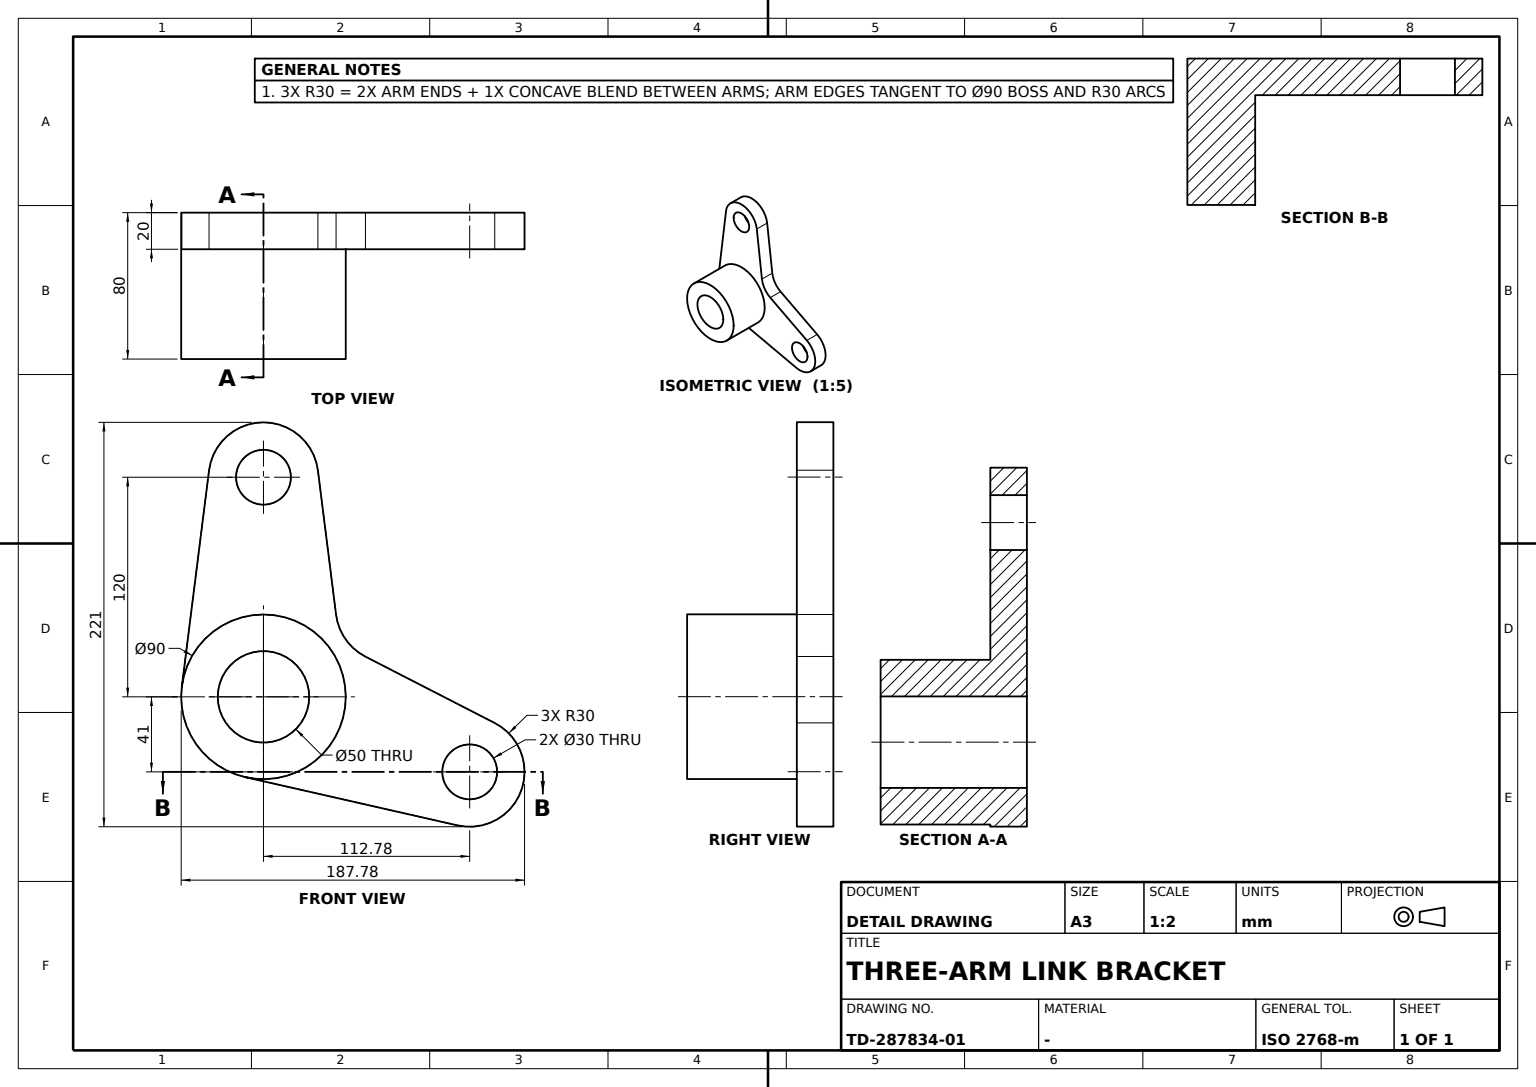
ISO-10303-21;
HEADER;
FILE_DESCRIPTION((''),'2;1');
FILE_NAME('','',(''),(''),'','','');
FILE_SCHEMA(('AUTOMOTIVE_DESIGN'));
ENDSEC;
DATA;
#1=APPLICATION_CONTEXT('');
#2=PRODUCT_CONTEXT('',#1,'mechanical');
#3=PRODUCT('','','',(#2));
#4=PRODUCT_DEFINITION_FORMATION('','',#3);
#5=PRODUCT_DEFINITION_CONTEXT('',#1,'design');
#6=PRODUCT_DEFINITION('','',#4,#5);
#7=PRODUCT_DEFINITION_SHAPE('','',#6);
#8=(LENGTH_UNIT()NAMED_UNIT(*)SI_UNIT(.MILLI.,.METRE.));
#9=(NAMED_UNIT(*)PLANE_ANGLE_UNIT()SI_UNIT($,.RADIAN.));
#10=(NAMED_UNIT(*)SI_UNIT($,.STERADIAN.)SOLID_ANGLE_UNIT());
#11=UNCERTAINTY_MEASURE_WITH_UNIT(LENGTH_MEASURE(1.E-05),#8,'distance_accuracy_value','');
#12=(GEOMETRIC_REPRESENTATION_CONTEXT(3)GLOBAL_UNCERTAINTY_ASSIGNED_CONTEXT((#11))GLOBAL_UNIT_ASSIGNED_CONTEXT((#8,#9,#10))REPRESENTATION_CONTEXT('',''));
#13=CARTESIAN_POINT('',(20.,45.,0.));
#14=VERTEX_POINT('',#13);
#15=CARTESIAN_POINT('',(20.,-44.647053,5.625));
#16=VERTEX_POINT('',#15);
#17=CARTESIAN_POINT('',(20.,0.,0.));
#18=DIRECTION('',(1.,0.,0.));
#19=DIRECTION('',(0.,1.,0.));
#20=AXIS2_PLACEMENT_3D('',#17,#18,#19);
#21=CIRCLE('',#20,45.);
#22=EDGE_CURVE('',#14,#16,#21,.T.);
#23=ORIENTED_EDGE('',*,*,#22,.T.);
#24=CARTESIAN_POINT('',(80.,-44.647053,5.625));
#25=VERTEX_POINT('',#24);
#26=CARTESIAN_POINT('',(40.,-44.647053,5.625));
#27=VECTOR('',#18,1000.);
#28=LINE('',#26,#27);
#29=EDGE_CURVE('',#16,#25,#28,.T.);
#30=ORIENTED_EDGE('',*,*,#29,.T.);
#31=CARTESIAN_POINT('',(80.,45.,0.));
#32=VERTEX_POINT('',#31);
#33=CARTESIAN_POINT('',(80.,0.,0.));
#34=AXIS2_PLACEMENT_3D('',#33,#18,#19);
#35=CIRCLE('',#34,45.);
#36=EDGE_CURVE('',#32,#25,#35,.T.);
#37=ORIENTED_EDGE('',*,*,#36,.F.);
#38=CARTESIAN_POINT('',(40.,45.,0.));
#39=DIRECTION('',(-1.,0.,0.));
#40=VECTOR('',#39,1000.);
#41=LINE('',#38,#40);
#42=EDGE_CURVE('',#32,#14,#41,.T.);
#43=ORIENTED_EDGE('',*,*,#42,.T.);
#44=EDGE_LOOP('',(#23,#30,#37,#43));
#45=FACE_OUTER_BOUND('',#44,.T.);
#46=CARTESIAN_POINT('',(40.,0.,0.));
#47=AXIS2_PLACEMENT_3D('',#46,#39,#19);
#48=CYLINDRICAL_SURFACE('',#47,45.);
#49=ADVANCED_FACE('',(#45),#48,.T.);
#50=CARTESIAN_POINT('',(0.,-29.764702,123.75));
#51=VERTEX_POINT('',#50);
#52=CARTESIAN_POINT('',(20.,-29.764702,123.75));
#53=VERTEX_POINT('',#52);
#54=CARTESIAN_POINT('',(10.,-29.764702,123.75));
#55=LINE('',#54,#27);
#56=EDGE_CURVE('',#51,#53,#55,.T.);
#57=ORIENTED_EDGE('',*,*,#56,.F.);
#58=CARTESIAN_POINT('',(0.,-44.647053,5.625));
#59=VERTEX_POINT('',#58);
#60=CARTESIAN_POINT('',(0.,-37.205878,64.6875));
#61=DIRECTION('',(0.,-0.125,-0.992156742));
#62=VECTOR('',#61,1000.);
#63=LINE('',#60,#62);
#64=EDGE_CURVE('',#51,#59,#63,.T.);
#65=ORIENTED_EDGE('',*,*,#64,.T.);
#66=CARTESIAN_POINT('',(10.,-44.647053,5.625));
#67=LINE('',#66,#27);
#68=EDGE_CURVE('',#59,#16,#67,.T.);
#69=ORIENTED_EDGE('',*,*,#68,.T.);
#70=CARTESIAN_POINT('',(20.,-37.205878,64.6875));
#71=LINE('',#70,#62);
#72=EDGE_CURVE('',#53,#16,#71,.T.);
#73=ORIENTED_EDGE('',*,*,#72,.F.);
#74=EDGE_LOOP('',(#57,#65,#69,#73));
#75=FACE_OUTER_BOUND('',#74,.T.);
#76=DIRECTION('',(0.,-0.992156742,0.125));
#77=AXIS2_PLACEMENT_3D('',#50,#76,#61);
#78=PLANE('',#77);
#79=ADVANCED_FACE('',(#75),#78,.T.);
#80=CARTESIAN_POINT('',(0.,142.778544,-41.));
#81=VERTEX_POINT('',#80);
#82=CARTESIAN_POINT('',(0.,126.47248,-14.307752));
#83=VERTEX_POINT('',#82);
#84=CARTESIAN_POINT('',(0.,112.778544,-41.));
#85=AXIS2_PLACEMENT_3D('',#84,#18,#19);
#86=CIRCLE('',#85,30.);
#87=EDGE_CURVE('',#81,#83,#86,.T.);
#88=ORIENTED_EDGE('',*,*,#87,.T.);
#89=CARTESIAN_POINT('',(20.,126.47248,-14.307752));
#90=VERTEX_POINT('',#89);
#91=CARTESIAN_POINT('',(10.,126.47248,-14.307752));
#92=LINE('',#91,#27);
#93=EDGE_CURVE('',#83,#90,#92,.T.);
#94=ORIENTED_EDGE('',*,*,#93,.T.);
#95=CARTESIAN_POINT('',(20.,142.778544,-41.));
#96=VERTEX_POINT('',#95);
#97=CARTESIAN_POINT('',(20.,112.778544,-41.));
#98=AXIS2_PLACEMENT_3D('',#97,#18,#19);
#99=CIRCLE('',#98,30.);
#100=EDGE_CURVE('',#96,#90,#99,.T.);
#101=ORIENTED_EDGE('',*,*,#100,.F.);
#102=CARTESIAN_POINT('',(10.,142.778544,-41.));
#103=LINE('',#102,#40);
#104=EDGE_CURVE('',#96,#81,#103,.T.);
#105=ORIENTED_EDGE('',*,*,#104,.T.);
#106=EDGE_LOOP('',(#88,#94,#101,#105));
#107=FACE_OUTER_BOUND('',#106,.T.);
#108=CARTESIAN_POINT('',(10.,112.778544,-41.));
#109=AXIS2_PLACEMENT_3D('',#108,#39,#19);
#110=CYLINDRICAL_SURFACE('',#109,30.);
#111=ADVANCED_FACE('',(#107),#110,.T.);
#112=CARTESIAN_POINT('',(0.,106.133267,-70.254748));
#113=VERTEX_POINT('',#112);
#114=CARTESIAN_POINT('',(20.,106.133267,-70.254748));
#115=VERTEX_POINT('',#114);
#116=CARTESIAN_POINT('',(10.,106.133267,-70.254748));
#117=LINE('',#116,#27);
#118=EDGE_CURVE('',#113,#115,#117,.T.);
#119=ORIENTED_EDGE('',*,*,#118,.T.);
#120=CARTESIAN_POINT('',(20.,-9.967916,-43.882122));
#121=VERTEX_POINT('',#120);
#122=CARTESIAN_POINT('',(20.,48.082676,-57.068435));
#123=DIRECTION('',(0.,0.975158273,-0.221509237));
#124=VECTOR('',#123,1000.);
#125=LINE('',#122,#124);
#126=EDGE_CURVE('',#121,#115,#125,.T.);
#127=ORIENTED_EDGE('',*,*,#126,.F.);
#128=CARTESIAN_POINT('',(0.,-9.967916,-43.882122));
#129=VERTEX_POINT('',#128);
#130=CARTESIAN_POINT('',(10.,-9.967916,-43.882122));
#131=LINE('',#130,#27);
#132=EDGE_CURVE('',#129,#121,#131,.T.);
#133=ORIENTED_EDGE('',*,*,#132,.F.);
#134=CARTESIAN_POINT('',(0.,48.082676,-57.068435));
#135=LINE('',#134,#124);
#136=EDGE_CURVE('',#129,#113,#135,.T.);
#137=ORIENTED_EDGE('',*,*,#136,.T.);
#138=EDGE_LOOP('',(#119,#127,#133,#137));
#139=FACE_OUTER_BOUND('',#138,.T.);
#140=DIRECTION('',(0.,-0.221509237,-0.975158273));
#141=AXIS2_PLACEMENT_3D('',#128,#140,#123);
#142=PLANE('',#141);
#143=ADVANCED_FACE('',(#139),#142,.T.);
#144=CARTESIAN_POINT('',(0.,15.,120.));
#145=VERTEX_POINT('',#144);
#146=CARTESIAN_POINT('',(0.,-15.,120.));
#147=VERTEX_POINT('',#146);
#148=CARTESIAN_POINT('',(0.,0.,120.));
#149=AXIS2_PLACEMENT_3D('',#148,#18,#19);
#150=CIRCLE('',#149,15.);
#151=EDGE_CURVE('',#145,#147,#150,.T.);
#152=ORIENTED_EDGE('',*,*,#151,.F.);
#153=CARTESIAN_POINT('',(20.,15.,120.));
#154=VERTEX_POINT('',#153);
#155=CARTESIAN_POINT('',(10.,15.,120.));
#156=LINE('',#155,#27);
#157=EDGE_CURVE('',#145,#154,#156,.T.);
#158=ORIENTED_EDGE('',*,*,#157,.T.);
#159=CARTESIAN_POINT('',(20.,-15.,120.));
#160=VERTEX_POINT('',#159);
#161=CARTESIAN_POINT('',(20.,0.,120.));
#162=AXIS2_PLACEMENT_3D('',#161,#18,#19);
#163=CIRCLE('',#162,15.);
#164=EDGE_CURVE('',#154,#160,#163,.T.);
#165=ORIENTED_EDGE('',*,*,#164,.T.);
#166=CARTESIAN_POINT('',(10.,-15.,120.));
#167=LINE('',#166,#27);
#168=EDGE_CURVE('',#147,#160,#167,.T.);
#169=ORIENTED_EDGE('',*,*,#168,.F.);
#170=EDGE_LOOP('',(#152,#158,#165,#169));
#171=FACE_OUTER_BOUND('',#170,.T.);
#172=CARTESIAN_POINT('',(10.,0.,120.));
#173=AXIS2_PLACEMENT_3D('',#172,#39,#19);
#174=CYLINDRICAL_SURFACE('',#173,15.);
#175=ADVANCED_FACE('',(#171),#174,.F.);
#176=CARTESIAN_POINT('',(0.,97.778544,-41.));
#177=VERTEX_POINT('',#176);
#178=CARTESIAN_POINT('',(0.,127.778544,-41.));
#179=VERTEX_POINT('',#178);
#180=CIRCLE('',#85,15.);
#181=EDGE_CURVE('',#177,#179,#180,.T.);
#182=ORIENTED_EDGE('',*,*,#181,.T.);
#183=EDGE_CURVE('',#179,#177,#180,.T.);
#184=ORIENTED_EDGE('',*,*,#183,.T.);
#185=EDGE_LOOP('',(#182,#184));
#186=FACE_BOUND('',#185,.T.);
#187=EDGE_CURVE('',#147,#145,#150,.T.);
#188=ORIENTED_EDGE('',*,*,#187,.T.);
#189=ORIENTED_EDGE('',*,*,#151,.T.);
#190=EDGE_LOOP('',(#188,#189));
#191=FACE_BOUND('',#190,.T.);
#192=CARTESIAN_POINT('',(0.,25.,0.));
#193=VERTEX_POINT('',#192);
#194=CARTESIAN_POINT('',(0.,-25.,0.));
#195=VERTEX_POINT('',#194);
#196=CARTESIAN_POINT('',(0.,0.,0.));
#197=AXIS2_PLACEMENT_3D('',#196,#18,#19);
#198=CIRCLE('',#197,25.);
#199=EDGE_CURVE('',#193,#195,#198,.T.);
#200=ORIENTED_EDGE('',*,*,#199,.T.);
#201=EDGE_CURVE('',#195,#193,#198,.T.);
#202=ORIENTED_EDGE('',*,*,#201,.T.);
#203=EDGE_LOOP('',(#200,#202));
#204=FACE_BOUND('',#203,.T.);
#205=CIRCLE('',#197,45.);
#206=EDGE_CURVE('',#59,#129,#205,.T.);
#207=ORIENTED_EDGE('',*,*,#206,.F.);
#208=ORIENTED_EDGE('',*,*,#64,.F.);
#209=CARTESIAN_POINT('',(0.,29.764702,123.75));
#210=VERTEX_POINT('',#209);
#211=CIRCLE('',#149,30.);
#212=EDGE_CURVE('',#210,#51,#211,.T.);
#213=ORIENTED_EDGE('',*,*,#212,.F.);
#214=CARTESIAN_POINT('',(0.,39.697897,44.907707));
#215=VERTEX_POINT('',#214);
#216=CARTESIAN_POINT('',(0.,34.7313,84.328854));
#217=DIRECTION('',(0.,0.125,-0.992156742));
#218=VECTOR('',#217,1000.);
#219=LINE('',#216,#218);
#220=EDGE_CURVE('',#210,#215,#219,.T.);
#221=ORIENTED_EDGE('',*,*,#220,.T.);
#222=CARTESIAN_POINT('',(0.,55.768664,21.965459));
#223=VERTEX_POINT('',#222);
#224=CARTESIAN_POINT('',(0.,69.4626,48.657707));
#225=AXIS2_PLACEMENT_3D('',#224,#18,#19);
#226=CIRCLE('',#225,30.);
#227=EDGE_CURVE('',#215,#223,#226,.T.);
#228=ORIENTED_EDGE('',*,*,#227,.T.);
#229=CARTESIAN_POINT('',(0.,91.120572,3.828854));
#230=DIRECTION('',(0.,0.889741607,-0.456464537));
#231=VECTOR('',#230,1000.);
#232=LINE('',#229,#231);
#233=EDGE_CURVE('',#223,#83,#232,.T.);
#234=ORIENTED_EDGE('',*,*,#233,.T.);
#235=ORIENTED_EDGE('',*,*,#87,.F.);
#236=EDGE_CURVE('',#113,#81,#86,.T.);
#237=ORIENTED_EDGE('',*,*,#236,.F.);
#238=ORIENTED_EDGE('',*,*,#136,.F.);
#239=EDGE_LOOP('',(#207,#208,#213,#221,#228,#234,#235,#237,#238));
#240=FACE_OUTER_BOUND('',#239,.T.);
#241=PLANE('',#197);
#242=ADVANCED_FACE('',(#186,#191,#204,#240),#241,.F.);
#243=ORIENTED_EDGE('',*,*,#56,.T.);
#244=CARTESIAN_POINT('',(20.,29.764702,123.75));
#245=VERTEX_POINT('',#244);
#246=CIRCLE('',#162,30.);
#247=EDGE_CURVE('',#245,#53,#246,.T.);
#248=ORIENTED_EDGE('',*,*,#247,.F.);
#249=CARTESIAN_POINT('',(10.,29.764702,123.75));
#250=LINE('',#249,#27);
#251=EDGE_CURVE('',#210,#245,#250,.T.);
#252=ORIENTED_EDGE('',*,*,#251,.F.);
#253=ORIENTED_EDGE('',*,*,#212,.T.);
#254=EDGE_LOOP('',(#243,#248,#252,#253));
#255=FACE_OUTER_BOUND('',#254,.T.);
#256=CYLINDRICAL_SURFACE('',#173,30.);
#257=ADVANCED_FACE('',(#255),#256,.T.);
#258=CARTESIAN_POINT('',(80.,-25.,0.));
#259=VERTEX_POINT('',#258);
#260=CARTESIAN_POINT('',(80.,25.,0.));
#261=VERTEX_POINT('',#260);
#262=CIRCLE('',#34,25.);
#263=EDGE_CURVE('',#259,#261,#262,.T.);
#264=ORIENTED_EDGE('',*,*,#263,.T.);
#265=CARTESIAN_POINT('',(39.34,25.,0.));
#266=LINE('',#265,#40);
#267=EDGE_CURVE('',#261,#193,#266,.T.);
#268=ORIENTED_EDGE('',*,*,#267,.T.);
#269=ORIENTED_EDGE('',*,*,#201,.F.);
#270=CARTESIAN_POINT('',(39.34,-25.,0.));
#271=LINE('',#270,#40);
#272=EDGE_CURVE('',#259,#195,#271,.T.);
#273=ORIENTED_EDGE('',*,*,#272,.F.);
#274=EDGE_LOOP('',(#264,#268,#269,#273));
#275=FACE_OUTER_BOUND('',#274,.T.);
#276=CARTESIAN_POINT('',(39.34,0.,0.));
#277=AXIS2_PLACEMENT_3D('',#276,#39,#19);
#278=CYLINDRICAL_SURFACE('',#277,25.);
#279=ADVANCED_FACE('',(#275),#278,.F.);
#280=ORIENTED_EDGE('',*,*,#263,.F.);
#281=EDGE_CURVE('',#261,#259,#262,.T.);
#282=ORIENTED_EDGE('',*,*,#281,.F.);
#283=EDGE_LOOP('',(#280,#282));
#284=FACE_BOUND('',#283,.T.);
#285=ORIENTED_EDGE('',*,*,#36,.T.);
#286=CARTESIAN_POINT('',(80.,-9.967916,-43.882122));
#287=VERTEX_POINT('',#286);
#288=EDGE_CURVE('',#25,#287,#35,.T.);
#289=ORIENTED_EDGE('',*,*,#288,.T.);
#290=EDGE_CURVE('',#287,#32,#35,.T.);
#291=ORIENTED_EDGE('',*,*,#290,.T.);
#292=EDGE_LOOP('',(#285,#289,#291));
#293=FACE_OUTER_BOUND('',#292,.T.);
#294=PLANE('',#34);
#295=ADVANCED_FACE('',(#284,#293),#294,.T.);
#296=CARTESIAN_POINT('',(20.,39.697897,44.907707));
#297=VERTEX_POINT('',#296);
#298=CARTESIAN_POINT('',(10.,39.697897,44.907707));
#299=LINE('',#298,#27);
#300=EDGE_CURVE('',#215,#297,#299,.T.);
#301=ORIENTED_EDGE('',*,*,#300,.T.);
#302=CARTESIAN_POINT('',(20.,55.768664,21.965459));
#303=VERTEX_POINT('',#302);
#304=CARTESIAN_POINT('',(20.,69.4626,48.657707));
#305=AXIS2_PLACEMENT_3D('',#304,#18,#19);
#306=CIRCLE('',#305,30.);
#307=EDGE_CURVE('',#297,#303,#306,.T.);
#308=ORIENTED_EDGE('',*,*,#307,.T.);
#309=CARTESIAN_POINT('',(10.,55.768664,21.965459));
#310=LINE('',#309,#27);
#311=EDGE_CURVE('',#223,#303,#310,.T.);
#312=ORIENTED_EDGE('',*,*,#311,.F.);
#313=ORIENTED_EDGE('',*,*,#227,.F.);
#314=EDGE_LOOP('',(#301,#308,#312,#313));
#315=FACE_OUTER_BOUND('',#314,.T.);
#316=CARTESIAN_POINT('',(10.,69.4626,48.657707));
#317=AXIS2_PLACEMENT_3D('',#316,#39,#19);
#318=CYLINDRICAL_SURFACE('',#317,30.);
#319=ADVANCED_FACE('',(#315),#318,.F.);
#320=ORIENTED_EDGE('',*,*,#164,.F.);
#321=EDGE_CURVE('',#160,#154,#163,.T.);
#322=ORIENTED_EDGE('',*,*,#321,.F.);
#323=EDGE_LOOP('',(#320,#322));
#324=FACE_BOUND('',#323,.T.);
#325=CARTESIAN_POINT('',(20.,97.778544,-41.));
#326=VERTEX_POINT('',#325);
#327=CARTESIAN_POINT('',(20.,127.778544,-41.));
#328=VERTEX_POINT('',#327);
#329=CIRCLE('',#98,15.);
#330=EDGE_CURVE('',#326,#328,#329,.T.);
#331=ORIENTED_EDGE('',*,*,#330,.F.);
#332=EDGE_CURVE('',#328,#326,#329,.T.);
#333=ORIENTED_EDGE('',*,*,#332,.F.);
#334=EDGE_LOOP('',(#331,#333));
#335=FACE_BOUND('',#334,.T.);
#336=ORIENTED_EDGE('',*,*,#247,.T.);
#337=ORIENTED_EDGE('',*,*,#72,.T.);
#338=ORIENTED_EDGE('',*,*,#22,.F.);
#339=EDGE_CURVE('',#121,#14,#21,.T.);
#340=ORIENTED_EDGE('',*,*,#339,.F.);
#341=ORIENTED_EDGE('',*,*,#126,.T.);
#342=EDGE_CURVE('',#115,#96,#99,.T.);
#343=ORIENTED_EDGE('',*,*,#342,.T.);
#344=ORIENTED_EDGE('',*,*,#100,.T.);
#345=CARTESIAN_POINT('',(20.,91.120572,3.828854));
#346=LINE('',#345,#231);
#347=EDGE_CURVE('',#303,#90,#346,.T.);
#348=ORIENTED_EDGE('',*,*,#347,.F.);
#349=ORIENTED_EDGE('',*,*,#307,.F.);
#350=CARTESIAN_POINT('',(20.,34.7313,84.328854));
#351=LINE('',#350,#218);
#352=EDGE_CURVE('',#245,#297,#351,.T.);
#353=ORIENTED_EDGE('',*,*,#352,.F.);
#354=EDGE_LOOP('',(#336,#337,#338,#340,#341,#343,#344,#348,#349,#353));
#355=FACE_OUTER_BOUND('',#354,.T.);
#356=PLANE('',#20);
#357=ADVANCED_FACE('',(#324,#335,#355),#356,.T.);
#358=ORIENTED_EDGE('',*,*,#104,.F.);
#359=ORIENTED_EDGE('',*,*,#342,.F.);
#360=ORIENTED_EDGE('',*,*,#118,.F.);
#361=ORIENTED_EDGE('',*,*,#236,.T.);
#362=EDGE_LOOP('',(#358,#359,#360,#361));
#363=FACE_OUTER_BOUND('',#362,.T.);
#364=ADVANCED_FACE('',(#363),#110,.T.);
#365=CARTESIAN_POINT('',(40.,-9.967916,-43.882122));
#366=LINE('',#365,#27);
#367=EDGE_CURVE('',#121,#287,#366,.T.);
#368=ORIENTED_EDGE('',*,*,#367,.F.);
#369=ORIENTED_EDGE('',*,*,#339,.T.);
#370=ORIENTED_EDGE('',*,*,#42,.F.);
#371=ORIENTED_EDGE('',*,*,#290,.F.);
#372=EDGE_LOOP('',(#368,#369,#370,#371));
#373=FACE_OUTER_BOUND('',#372,.T.);
#374=ADVANCED_FACE('',(#373),#48,.T.);
#375=ORIENTED_EDGE('',*,*,#300,.F.);
#376=ORIENTED_EDGE('',*,*,#220,.F.);
#377=ORIENTED_EDGE('',*,*,#251,.T.);
#378=ORIENTED_EDGE('',*,*,#352,.T.);
#379=EDGE_LOOP('',(#375,#376,#377,#378));
#380=FACE_OUTER_BOUND('',#379,.T.);
#381=DIRECTION('',(0.,-0.992156742,-0.125));
#382=AXIS2_PLACEMENT_3D('',#209,#381,#217);
#383=PLANE('',#382);
#384=ADVANCED_FACE('',(#380),#383,.F.);
#385=ORIENTED_EDGE('',*,*,#347,.T.);
#386=ORIENTED_EDGE('',*,*,#93,.F.);
#387=ORIENTED_EDGE('',*,*,#233,.F.);
#388=ORIENTED_EDGE('',*,*,#311,.T.);
#389=EDGE_LOOP('',(#385,#386,#387,#388));
#390=FACE_OUTER_BOUND('',#389,.T.);
#391=DIRECTION('',(0.,-0.456464537,-0.889741607));
#392=AXIS2_PLACEMENT_3D('',#222,#391,#230);
#393=PLANE('',#392);
#394=ADVANCED_FACE('',(#390),#393,.F.);
#395=ORIENTED_EDGE('',*,*,#367,.T.);
#396=ORIENTED_EDGE('',*,*,#288,.F.);
#397=ORIENTED_EDGE('',*,*,#29,.F.);
#398=ORIENTED_EDGE('',*,*,#68,.F.);
#399=ORIENTED_EDGE('',*,*,#206,.T.);
#400=ORIENTED_EDGE('',*,*,#132,.T.);
#401=EDGE_LOOP('',(#395,#396,#397,#398,#399,#400));
#402=FACE_OUTER_BOUND('',#401,.T.);
#403=ADVANCED_FACE('',(#402),#48,.T.);
#404=ORIENTED_EDGE('',*,*,#168,.T.);
#405=ORIENTED_EDGE('',*,*,#321,.T.);
#406=ORIENTED_EDGE('',*,*,#157,.F.);
#407=ORIENTED_EDGE('',*,*,#187,.F.);
#408=EDGE_LOOP('',(#404,#405,#406,#407));
#409=FACE_OUTER_BOUND('',#408,.T.);
#410=ADVANCED_FACE('',(#409),#174,.F.);
#411=ORIENTED_EDGE('',*,*,#330,.T.);
#412=CARTESIAN_POINT('',(10.,127.778544,-41.));
#413=LINE('',#412,#27);
#414=EDGE_CURVE('',#179,#328,#413,.T.);
#415=ORIENTED_EDGE('',*,*,#414,.F.);
#416=ORIENTED_EDGE('',*,*,#181,.F.);
#417=CARTESIAN_POINT('',(10.,97.778544,-41.));
#418=LINE('',#417,#27);
#419=EDGE_CURVE('',#177,#326,#418,.T.);
#420=ORIENTED_EDGE('',*,*,#419,.T.);
#421=EDGE_LOOP('',(#411,#415,#416,#420));
#422=FACE_OUTER_BOUND('',#421,.T.);
#423=CYLINDRICAL_SURFACE('',#109,15.);
#424=ADVANCED_FACE('',(#422),#423,.F.);
#425=ORIENTED_EDGE('',*,*,#183,.F.);
#426=ORIENTED_EDGE('',*,*,#414,.T.);
#427=ORIENTED_EDGE('',*,*,#332,.T.);
#428=ORIENTED_EDGE('',*,*,#419,.F.);
#429=EDGE_LOOP('',(#425,#426,#427,#428));
#430=FACE_OUTER_BOUND('',#429,.T.);
#431=ADVANCED_FACE('',(#430),#423,.F.);
#432=ORIENTED_EDGE('',*,*,#272,.T.);
#433=ORIENTED_EDGE('',*,*,#199,.F.);
#434=ORIENTED_EDGE('',*,*,#267,.F.);
#435=ORIENTED_EDGE('',*,*,#281,.T.);
#436=EDGE_LOOP('',(#432,#433,#434,#435));
#437=FACE_OUTER_BOUND('',#436,.T.);
#438=ADVANCED_FACE('',(#437),#278,.F.);
#439=CLOSED_SHELL('',(#49,#79,#111,#143,#175,#242,#257,#279,#295,#319,#357,#364,#374,#384,#394,#403,#410,#424,#431,#438));
#440=MANIFOLD_SOLID_BREP('',#439);
#441=ADVANCED_BREP_SHAPE_REPRESENTATION('',(#440),#12);
#442=SHAPE_DEFINITION_REPRESENTATION(#7,#441);
ENDSEC;
END-ISO-10303-21;
